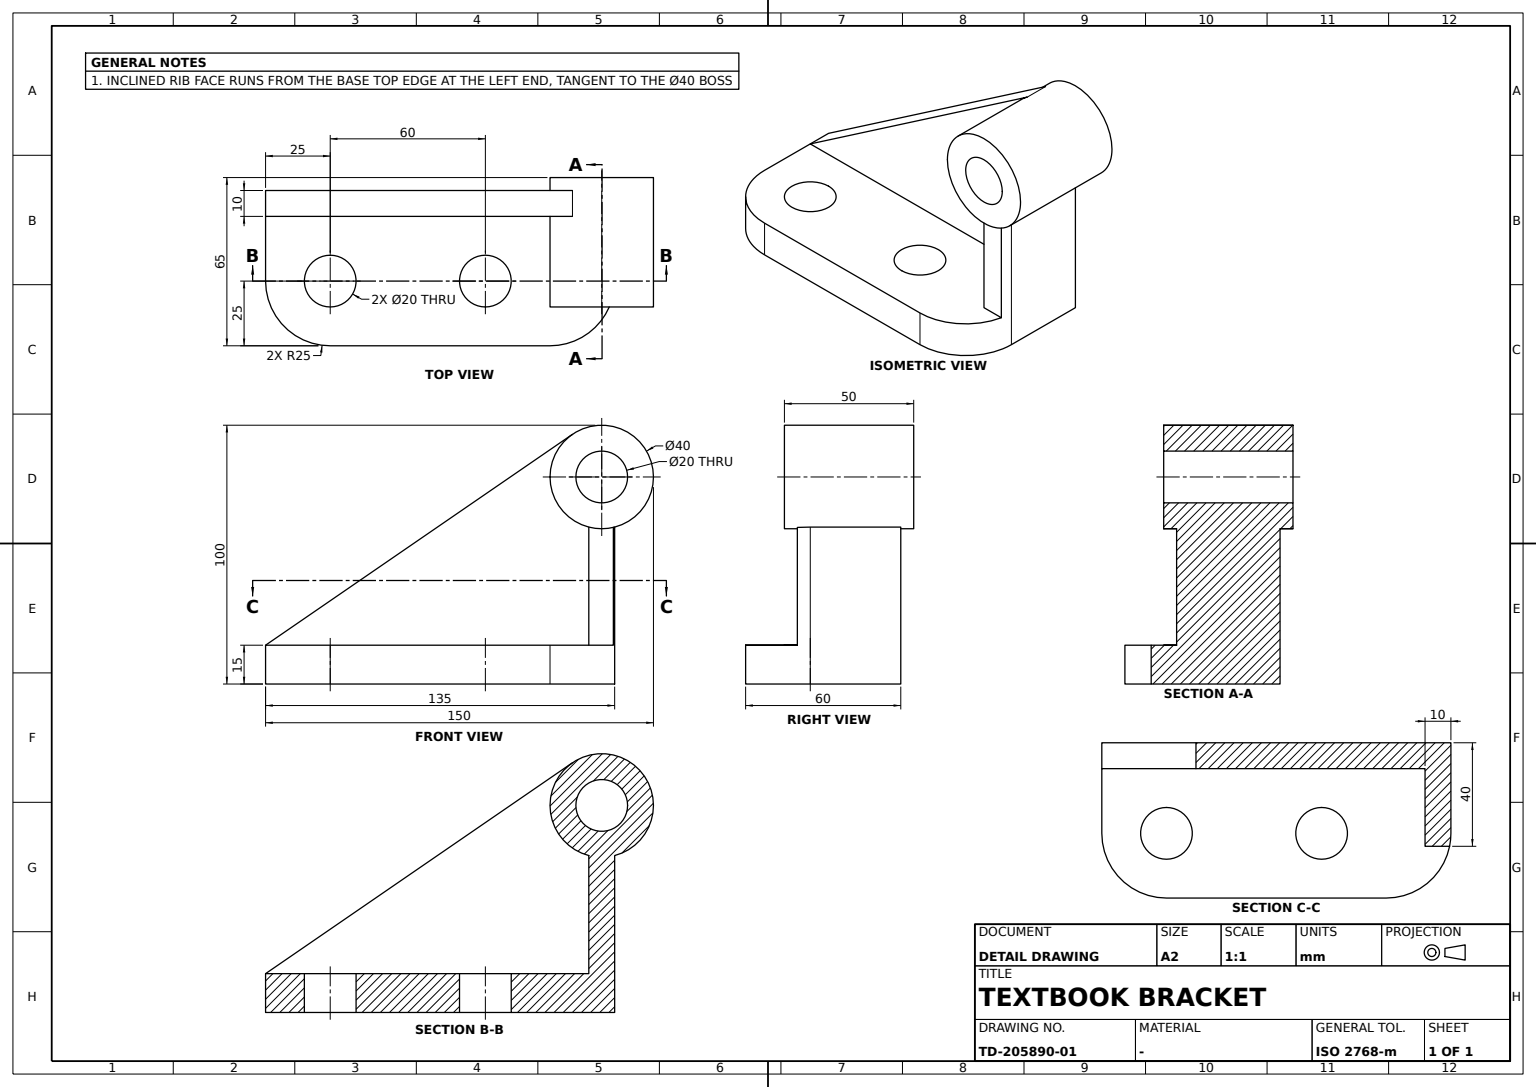
ISO-10303-21;
HEADER;
FILE_DESCRIPTION((''),'2;1');
FILE_NAME('','',(''),(''),'','','');
FILE_SCHEMA(('AUTOMOTIVE_DESIGN'));
ENDSEC;
DATA;
#1=APPLICATION_CONTEXT('');
#2=PRODUCT_CONTEXT('',#1,'mechanical');
#3=PRODUCT('','','',(#2));
#4=PRODUCT_DEFINITION_FORMATION('','',#3);
#5=PRODUCT_DEFINITION_CONTEXT('',#1,'design');
#6=PRODUCT_DEFINITION('','',#4,#5);
#7=PRODUCT_DEFINITION_SHAPE('','',#6);
#8=(LENGTH_UNIT()NAMED_UNIT(*)SI_UNIT(.MILLI.,.METRE.));
#9=(NAMED_UNIT(*)PLANE_ANGLE_UNIT()SI_UNIT($,.RADIAN.));
#10=(NAMED_UNIT(*)SI_UNIT($,.STERADIAN.)SOLID_ANGLE_UNIT());
#11=UNCERTAINTY_MEASURE_WITH_UNIT(LENGTH_MEASURE(1.E-05),#8,'distance_accuracy_value','');
#12=(GEOMETRIC_REPRESENTATION_CONTEXT(3)GLOBAL_UNCERTAINTY_ASSIGNED_CONTEXT((#11))GLOBAL_UNIT_ASSIGNED_CONTEXT((#8,#9,#10))REPRESENTATION_CONTEXT('',''));
#13=CARTESIAN_POINT('',(10.,55.,80.));
#14=VERTEX_POINT('',#13);
#15=CARTESIAN_POINT('',(10.,70.,60.635083));
#16=VERTEX_POINT('',#15);
#17=CARTESIAN_POINT('',(10.,75.,80.));
#18=DIRECTION('',(1.,0.,0.));
#19=DIRECTION('',(0.,1.,0.));
#20=AXIS2_PLACEMENT_3D('',#17,#18,#19);
#21=CIRCLE('',#20,20.);
#22=EDGE_CURVE('',#14,#16,#21,.T.);
#23=ORIENTED_EDGE('',*,*,#22,.T.);
#24=CARTESIAN_POINT('',(10.,80.,60.635083));
#25=VERTEX_POINT('',#24);
#26=EDGE_CURVE('',#16,#25,#21,.T.);
#27=ORIENTED_EDGE('',*,*,#26,.T.);
#28=CARTESIAN_POINT('',(10.,95.,80.));
#29=VERTEX_POINT('',#28);
#30=EDGE_CURVE('',#25,#29,#21,.T.);
#31=ORIENTED_EDGE('',*,*,#30,.T.);
#32=EDGE_CURVE('',#29,#14,#21,.T.);
#33=ORIENTED_EDGE('',*,*,#32,.T.);
#34=EDGE_LOOP('',(#23,#27,#31,#33));
#35=FACE_OUTER_BOUND('',#34,.T.);
#36=CARTESIAN_POINT('',(10.,85.,80.));
#37=VERTEX_POINT('',#36);
#38=CARTESIAN_POINT('',(10.,65.,80.));
#39=VERTEX_POINT('',#38);
#40=CIRCLE('',#20,10.);
#41=EDGE_CURVE('',#37,#39,#40,.T.);
#42=ORIENTED_EDGE('',*,*,#41,.F.);
#43=EDGE_CURVE('',#39,#37,#40,.T.);
#44=ORIENTED_EDGE('',*,*,#43,.F.);
#45=EDGE_LOOP('',(#42,#44));
#46=FACE_BOUND('',#45,.T.);
#47=CARTESIAN_POINT('',(10.,0.,0.));
#48=AXIS2_PLACEMENT_3D('',#47,#18,#19);
#49=PLANE('',#48);
#50=ADVANCED_FACE('',(#35,#46),#49,.T.);
#51=CARTESIAN_POINT('',(-35.,55.,80.));
#52=VERTEX_POINT('',#51);
#53=CARTESIAN_POINT('',(-40.,55.,80.));
#54=VERTEX_POINT('',#53);
#55=CARTESIAN_POINT('',(-15.,55.,80.));
#56=DIRECTION('',(-1.,0.,0.));
#57=VECTOR('',#56,1000.);
#58=LINE('',#55,#57);
#59=EDGE_CURVE('',#52,#54,#58,.T.);
#60=ORIENTED_EDGE('',*,*,#59,.F.);
#61=CARTESIAN_POINT('',(-35.,63.679274,96.487606));
#62=VERTEX_POINT('',#61);
#63=CARTESIAN_POINT('',(-35.,75.,80.));
#64=AXIS2_PLACEMENT_3D('',#63,#18,#19);
#65=CIRCLE('',#64,20.);
#66=EDGE_CURVE('',#62,#52,#65,.T.);
#67=ORIENTED_EDGE('',*,*,#66,.F.);
#68=CARTESIAN_POINT('',(-25.,63.679274,96.487606));
#69=VERTEX_POINT('',#68);
#70=CARTESIAN_POINT('',(-15.,63.679274,96.487606));
#71=VECTOR('',#18,1000.);
#72=LINE('',#70,#71);
#73=EDGE_CURVE('',#62,#69,#72,.T.);
#74=ORIENTED_EDGE('',*,*,#73,.T.);
#75=CARTESIAN_POINT('',(-25.,55.,80.));
#76=VERTEX_POINT('',#75);
#77=CARTESIAN_POINT('',(-25.,75.,80.));
#78=AXIS2_PLACEMENT_3D('',#77,#18,#19);
#79=CIRCLE('',#78,20.);
#80=EDGE_CURVE('',#69,#76,#79,.T.);
#81=ORIENTED_EDGE('',*,*,#80,.T.);
#82=EDGE_CURVE('',#14,#76,#58,.T.);
#83=ORIENTED_EDGE('',*,*,#82,.F.);
#84=ORIENTED_EDGE('',*,*,#32,.F.);
#85=CARTESIAN_POINT('',(-40.,95.,80.));
#86=VERTEX_POINT('',#85);
#87=CARTESIAN_POINT('',(-15.,95.,80.));
#88=LINE('',#87,#57);
#89=EDGE_CURVE('',#29,#86,#88,.T.);
#90=ORIENTED_EDGE('',*,*,#89,.T.);
#91=CARTESIAN_POINT('',(-40.,75.,80.));
#92=AXIS2_PLACEMENT_3D('',#91,#18,#19);
#93=CIRCLE('',#92,20.);
#94=EDGE_CURVE('',#86,#54,#93,.T.);
#95=ORIENTED_EDGE('',*,*,#94,.T.);
#96=EDGE_LOOP('',(#60,#67,#74,#81,#83,#84,#90,#95));
#97=FACE_OUTER_BOUND('',#96,.T.);
#98=CARTESIAN_POINT('',(-15.,75.,80.));
#99=AXIS2_PLACEMENT_3D('',#98,#56,#19);
#100=CYLINDRICAL_SURFACE('',#99,20.);
#101=ADVANCED_FACE('',(#97),#100,.T.);
#102=CARTESIAN_POINT('',(0.,-55.,0.));
#103=VERTEX_POINT('',#102);
#104=CARTESIAN_POINT('',(25.,-30.,0.));
#105=VERTEX_POINT('',#104);
#106=CARTESIAN_POINT('',(0.,-30.,0.));
#107=DIRECTION('',(0.,0.,1.));
#108=AXIS2_PLACEMENT_3D('',#106,#107,#56);
#109=CIRCLE('',#108,25.);
#110=EDGE_CURVE('',#103,#105,#109,.T.);
#111=ORIENTED_EDGE('',*,*,#110,.T.);
#112=CARTESIAN_POINT('',(25.,-30.,15.));
#113=VERTEX_POINT('',#112);
#114=CARTESIAN_POINT('',(25.,-30.,7.5));
#115=VECTOR('',#107,1000.);
#116=LINE('',#114,#115);
#117=EDGE_CURVE('',#105,#113,#116,.T.);
#118=ORIENTED_EDGE('',*,*,#117,.T.);
#119=CARTESIAN_POINT('',(0.,-55.,15.));
#120=VERTEX_POINT('',#119);
#121=CARTESIAN_POINT('',(0.,-30.,15.));
#122=DIRECTION('',(0.,0.,-1.));
#123=AXIS2_PLACEMENT_3D('',#121,#122,#56);
#124=CIRCLE('',#123,25.);
#125=EDGE_CURVE('',#113,#120,#124,.T.);
#126=ORIENTED_EDGE('',*,*,#125,.T.);
#127=CARTESIAN_POINT('',(0.,-55.,7.5));
#128=LINE('',#127,#115);
#129=EDGE_CURVE('',#103,#120,#128,.T.);
#130=ORIENTED_EDGE('',*,*,#129,.F.);
#131=EDGE_LOOP('',(#111,#118,#126,#130));
#132=FACE_OUTER_BOUND('',#131,.T.);
#133=CARTESIAN_POINT('',(0.,-30.,7.5));
#134=AXIS2_PLACEMENT_3D('',#133,#122,#18);
#135=CYLINDRICAL_SURFACE('',#134,25.);
#136=ADVANCED_FACE('',(#132),#135,.T.);
#137=CARTESIAN_POINT('',(-40.,65.,80.));
#138=VERTEX_POINT('',#137);
#139=CARTESIAN_POINT('',(-40.,85.,80.));
#140=VERTEX_POINT('',#139);
#141=CIRCLE('',#92,10.);
#142=EDGE_CURVE('',#138,#140,#141,.T.);
#143=ORIENTED_EDGE('',*,*,#142,.F.);
#144=CARTESIAN_POINT('',(-15.,65.,80.));
#145=LINE('',#144,#71);
#146=EDGE_CURVE('',#138,#39,#145,.T.);
#147=ORIENTED_EDGE('',*,*,#146,.T.);
#148=ORIENTED_EDGE('',*,*,#43,.T.);
#149=CARTESIAN_POINT('',(-15.,85.,80.));
#150=LINE('',#149,#71);
#151=EDGE_CURVE('',#140,#37,#150,.T.);
#152=ORIENTED_EDGE('',*,*,#151,.F.);
#153=EDGE_LOOP('',(#143,#147,#148,#152));
#154=FACE_OUTER_BOUND('',#153,.T.);
#155=CYLINDRICAL_SURFACE('',#99,10.);
#156=ADVANCED_FACE('',(#154),#155,.F.);
#157=CARTESIAN_POINT('',(5.,70.,15.));
#158=VERTEX_POINT('',#157);
#159=CARTESIAN_POINT('',(5.,79.494897,15.));
#160=VERTEX_POINT('',#159);
#161=CARTESIAN_POINT('',(5.,74.747449,15.));
#162=VECTOR('',#19,1000.);
#163=LINE('',#161,#162);
#164=EDGE_CURVE('',#158,#160,#163,.T.);
#165=ORIENTED_EDGE('',*,*,#164,.T.);
#166=CARTESIAN_POINT('',(5.,79.494897,60.511647));
#167=VERTEX_POINT('',#166);
#168=CARTESIAN_POINT('',(5.,79.494897,37.755824));
#169=VECTOR('',#122,1000.);
#170=LINE('',#168,#169);
#171=EDGE_CURVE('',#167,#160,#170,.T.);
#172=ORIENTED_EDGE('',*,*,#171,.F.);
#173=CARTESIAN_POINT('',(5.,70.,60.635083));
#174=VERTEX_POINT('',#173);
#175=CARTESIAN_POINT('',(5.,75.,80.));
#176=AXIS2_PLACEMENT_3D('',#175,#18,#19);
#177=CIRCLE('',#176,20.);
#178=EDGE_CURVE('',#174,#167,#177,.T.);
#179=ORIENTED_EDGE('',*,*,#178,.F.);
#180=CARTESIAN_POINT('',(5.,70.,37.817542));
#181=LINE('',#180,#169);
#182=EDGE_CURVE('',#174,#158,#181,.T.);
#183=ORIENTED_EDGE('',*,*,#182,.T.);
#184=EDGE_LOOP('',(#165,#172,#179,#183));
#185=FACE_OUTER_BOUND('',#184,.T.);
#186=CARTESIAN_POINT('',(5.,0.,0.));
#187=AXIS2_PLACEMENT_3D('',#186,#18,#19);
#188=PLANE('',#187);
#189=ADVANCED_FACE('',(#185),#188,.T.);
#190=CARTESIAN_POINT('',(-35.,-55.,15.));
#191=VERTEX_POINT('',#190);
#192=CARTESIAN_POINT('',(-35.,4.339637,55.743803));
#193=DIRECTION('',(0.,-0.824380311,-0.566036309));
#194=VECTOR('',#193,1000.);
#195=LINE('',#192,#194);
#196=EDGE_CURVE('',#62,#191,#195,.T.);
#197=ORIENTED_EDGE('',*,*,#196,.T.);
#198=CARTESIAN_POINT('',(-25.,-55.,15.));
#199=VERTEX_POINT('',#198);
#200=CARTESIAN_POINT('',(-30.,-55.,15.));
#201=LINE('',#200,#71);
#202=EDGE_CURVE('',#191,#199,#201,.T.);
#203=ORIENTED_EDGE('',*,*,#202,.T.);
#204=CARTESIAN_POINT('',(-25.,4.339637,55.743803));
#205=LINE('',#204,#194);
#206=EDGE_CURVE('',#69,#199,#205,.T.);
#207=ORIENTED_EDGE('',*,*,#206,.F.);
#208=ORIENTED_EDGE('',*,*,#73,.F.);
#209=EDGE_LOOP('',(#197,#203,#207,#208));
#210=FACE_OUTER_BOUND('',#209,.T.);
#211=DIRECTION('',(0.,0.566036309,-0.824380311));
#212=DIRECTION('',(0.,0.824380311,0.566036309));
#213=AXIS2_PLACEMENT_3D('',#61,#211,#212);
#214=PLANE('',#213);
#215=ADVANCED_FACE('',(#210),#214,.F.);
#216=ORIENTED_EDGE('',*,*,#66,.T.);
#217=CARTESIAN_POINT('',(-35.,70.,60.635083));
#218=VERTEX_POINT('',#217);
#219=EDGE_CURVE('',#52,#218,#65,.T.);
#220=ORIENTED_EDGE('',*,*,#219,.T.);
#221=CARTESIAN_POINT('',(-35.,80.,60.635083));
#222=VERTEX_POINT('',#221);
#223=EDGE_CURVE('',#218,#222,#65,.T.);
#224=ORIENTED_EDGE('',*,*,#223,.T.);
#225=CARTESIAN_POINT('',(-35.,80.,0.));
#226=VERTEX_POINT('',#225);
#227=CARTESIAN_POINT('',(-35.,80.,30.317542));
#228=LINE('',#227,#115);
#229=EDGE_CURVE('',#226,#222,#228,.T.);
#230=ORIENTED_EDGE('',*,*,#229,.F.);
#231=CARTESIAN_POINT('',(-35.,-55.,0.));
#232=VERTEX_POINT('',#231);
#233=CARTESIAN_POINT('',(-35.,12.5,0.));
#234=DIRECTION('',(0.,-1.,0.));
#235=VECTOR('',#234,1000.);
#236=LINE('',#233,#235);
#237=EDGE_CURVE('',#226,#232,#236,.T.);
#238=ORIENTED_EDGE('',*,*,#237,.T.);
#239=CARTESIAN_POINT('',(-35.,-55.,7.5));
#240=LINE('',#239,#169);
#241=EDGE_CURVE('',#191,#232,#240,.T.);
#242=ORIENTED_EDGE('',*,*,#241,.F.);
#243=ORIENTED_EDGE('',*,*,#196,.F.);
#244=EDGE_LOOP('',(#216,#220,#224,#230,#238,#242,#243));
#245=FACE_OUTER_BOUND('',#244,.T.);
#246=CARTESIAN_POINT('',(-35.,0.,0.));
#247=AXIS2_PLACEMENT_3D('',#246,#18,#19);
#248=PLANE('',#247);
#249=ADVANCED_FACE('',(#245),#248,.F.);
#250=CARTESIAN_POINT('',(10.,30.,0.));
#251=VERTEX_POINT('',#250);
#252=CARTESIAN_POINT('',(-10.,30.,0.));
#253=VERTEX_POINT('',#252);
#254=CARTESIAN_POINT('',(0.,30.,0.));
#255=AXIS2_PLACEMENT_3D('',#254,#107,#56);
#256=CIRCLE('',#255,10.);
#257=EDGE_CURVE('',#251,#253,#256,.T.);
#258=ORIENTED_EDGE('',*,*,#257,.T.);
#259=EDGE_CURVE('',#253,#251,#256,.T.);
#260=ORIENTED_EDGE('',*,*,#259,.T.);
#261=EDGE_LOOP('',(#258,#260));
#262=FACE_BOUND('',#261,.T.);
#263=CARTESIAN_POINT('',(-17.5,-55.,0.));
#264=LINE('',#263,#71);
#265=EDGE_CURVE('',#232,#103,#264,.T.);
#266=ORIENTED_EDGE('',*,*,#265,.F.);
#267=ORIENTED_EDGE('',*,*,#237,.F.);
#268=CARTESIAN_POINT('',(0.,80.,0.));
#269=VERTEX_POINT('',#268);
#270=CARTESIAN_POINT('',(-17.5,80.,0.));
#271=LINE('',#270,#57);
#272=EDGE_CURVE('',#269,#226,#271,.T.);
#273=ORIENTED_EDGE('',*,*,#272,.F.);
#274=CARTESIAN_POINT('',(25.,55.,0.));
#275=VERTEX_POINT('',#274);
#276=CARTESIAN_POINT('',(0.,55.,0.));
#277=AXIS2_PLACEMENT_3D('',#276,#107,#56);
#278=CIRCLE('',#277,25.);
#279=EDGE_CURVE('',#275,#269,#278,.T.);
#280=ORIENTED_EDGE('',*,*,#279,.F.);
#281=CARTESIAN_POINT('',(25.,12.5,0.));
#282=LINE('',#281,#162);
#283=EDGE_CURVE('',#105,#275,#282,.T.);
#284=ORIENTED_EDGE('',*,*,#283,.F.);
#285=ORIENTED_EDGE('',*,*,#110,.F.);
#286=EDGE_LOOP('',(#266,#267,#273,#280,#284,#285));
#287=FACE_OUTER_BOUND('',#286,.T.);
#288=CARTESIAN_POINT('',(10.,-30.,0.));
#289=VERTEX_POINT('',#288);
#290=CARTESIAN_POINT('',(-10.,-30.,0.));
#291=VERTEX_POINT('',#290);
#292=CIRCLE('',#108,10.);
#293=EDGE_CURVE('',#289,#291,#292,.T.);
#294=ORIENTED_EDGE('',*,*,#293,.T.);
#295=EDGE_CURVE('',#291,#289,#292,.T.);
#296=ORIENTED_EDGE('',*,*,#295,.T.);
#297=EDGE_LOOP('',(#294,#296));
#298=FACE_BOUND('',#297,.T.);
#299=CARTESIAN_POINT('',(0.,0.,0.));
#300=AXIS2_PLACEMENT_3D('',#299,#107,#56);
#301=PLANE('',#300);
#302=ADVANCED_FACE('',(#262,#287,#298),#301,.F.);
#303=CARTESIAN_POINT('',(25.,55.,15.));
#304=VERTEX_POINT('',#303);
#305=CARTESIAN_POINT('',(25.,12.5,15.));
#306=LINE('',#305,#162);
#307=EDGE_CURVE('',#113,#304,#306,.T.);
#308=ORIENTED_EDGE('',*,*,#307,.F.);
#309=ORIENTED_EDGE('',*,*,#117,.F.);
#310=ORIENTED_EDGE('',*,*,#283,.T.);
#311=CARTESIAN_POINT('',(25.,55.,7.5));
#312=LINE('',#311,#115);
#313=EDGE_CURVE('',#275,#304,#312,.T.);
#314=ORIENTED_EDGE('',*,*,#313,.T.);
#315=EDGE_LOOP('',(#308,#309,#310,#314));
#316=FACE_OUTER_BOUND('',#315,.T.);
#317=CARTESIAN_POINT('',(25.,-55.,0.));
#318=AXIS2_PLACEMENT_3D('',#317,#18,#19);
#319=PLANE('',#318);
#320=ADVANCED_FACE('',(#316),#319,.T.);
#321=CARTESIAN_POINT('',(-10.,-30.,15.));
#322=VERTEX_POINT('',#321);
#323=CARTESIAN_POINT('',(10.,-30.,15.));
#324=VERTEX_POINT('',#323);
#325=AXIS2_PLACEMENT_3D('',#121,#107,#56);
#326=CIRCLE('',#325,10.);
#327=EDGE_CURVE('',#322,#324,#326,.T.);
#328=ORIENTED_EDGE('',*,*,#327,.T.);
#329=CARTESIAN_POINT('',(10.,-30.,7.5));
#330=LINE('',#329,#115);
#331=EDGE_CURVE('',#289,#324,#330,.T.);
#332=ORIENTED_EDGE('',*,*,#331,.F.);
#333=ORIENTED_EDGE('',*,*,#295,.F.);
#334=CARTESIAN_POINT('',(-10.,-30.,7.5));
#335=LINE('',#334,#115);
#336=EDGE_CURVE('',#291,#322,#335,.T.);
#337=ORIENTED_EDGE('',*,*,#336,.T.);
#338=EDGE_LOOP('',(#328,#332,#333,#337));
#339=FACE_OUTER_BOUND('',#338,.T.);
#340=AXIS2_PLACEMENT_3D('',#133,#122,#56);
#341=CYLINDRICAL_SURFACE('',#340,10.);
#342=ADVANCED_FACE('',(#339),#341,.F.);
#343=ORIENTED_EDGE('',*,*,#259,.F.);
#344=CARTESIAN_POINT('',(-10.,30.,15.));
#345=VERTEX_POINT('',#344);
#346=CARTESIAN_POINT('',(-10.,30.,7.5));
#347=LINE('',#346,#115);
#348=EDGE_CURVE('',#253,#345,#347,.T.);
#349=ORIENTED_EDGE('',*,*,#348,.T.);
#350=CARTESIAN_POINT('',(10.,30.,15.));
#351=VERTEX_POINT('',#350);
#352=CARTESIAN_POINT('',(0.,30.,15.));
#353=AXIS2_PLACEMENT_3D('',#352,#107,#56);
#354=CIRCLE('',#353,10.);
#355=EDGE_CURVE('',#345,#351,#354,.T.);
#356=ORIENTED_EDGE('',*,*,#355,.T.);
#357=CARTESIAN_POINT('',(10.,30.,7.5));
#358=LINE('',#357,#115);
#359=EDGE_CURVE('',#251,#351,#358,.T.);
#360=ORIENTED_EDGE('',*,*,#359,.F.);
#361=EDGE_LOOP('',(#343,#349,#356,#360));
#362=FACE_OUTER_BOUND('',#361,.T.);
#363=CARTESIAN_POINT('',(0.,30.,7.5));
#364=AXIS2_PLACEMENT_3D('',#363,#122,#56);
#365=CYLINDRICAL_SURFACE('',#364,10.);
#366=ADVANCED_FACE('',(#362),#365,.F.);
#367=CARTESIAN_POINT('',(-12.5,-55.,15.));
#368=LINE('',#367,#71);
#369=EDGE_CURVE('',#199,#120,#368,.T.);
#370=ORIENTED_EDGE('',*,*,#369,.F.);
#371=ORIENTED_EDGE('',*,*,#202,.F.);
#372=ORIENTED_EDGE('',*,*,#241,.T.);
#373=ORIENTED_EDGE('',*,*,#265,.T.);
#374=ORIENTED_EDGE('',*,*,#129,.T.);
#375=EDGE_LOOP('',(#370,#371,#372,#373,#374));
#376=FACE_OUTER_BOUND('',#375,.T.);
#377=CARTESIAN_POINT('',(-25.,-55.,0.));
#378=AXIS2_PLACEMENT_3D('',#377,#234,#18);
#379=PLANE('',#378);
#380=ADVANCED_FACE('',(#376),#379,.T.);
#381=CARTESIAN_POINT('',(-40.,70.,60.635083));
#382=VERTEX_POINT('',#381);
#383=CARTESIAN_POINT('',(-15.,70.,60.635083));
#384=LINE('',#383,#71);
#385=EDGE_CURVE('',#382,#218,#384,.T.);
#386=ORIENTED_EDGE('',*,*,#385,.T.);
#387=ORIENTED_EDGE('',*,*,#219,.F.);
#388=ORIENTED_EDGE('',*,*,#59,.T.);
#389=EDGE_CURVE('',#54,#382,#93,.T.);
#390=ORIENTED_EDGE('',*,*,#389,.T.);
#391=EDGE_LOOP('',(#386,#387,#388,#390));
#392=FACE_OUTER_BOUND('',#391,.T.);
#393=ADVANCED_FACE('',(#392),#100,.T.);
#394=ORIENTED_EDGE('',*,*,#331,.T.);
#395=EDGE_CURVE('',#324,#322,#326,.T.);
#396=ORIENTED_EDGE('',*,*,#395,.T.);
#397=ORIENTED_EDGE('',*,*,#336,.F.);
#398=ORIENTED_EDGE('',*,*,#293,.F.);
#399=EDGE_LOOP('',(#394,#396,#397,#398));
#400=FACE_OUTER_BOUND('',#399,.T.);
#401=ADVANCED_FACE('',(#400),#341,.F.);
#402=ORIENTED_EDGE('',*,*,#182,.F.);
#403=CARTESIAN_POINT('',(-25.,70.,60.635083));
#404=VERTEX_POINT('',#403);
#405=CARTESIAN_POINT('',(-10.,70.,60.635083));
#406=LINE('',#405,#71);
#407=EDGE_CURVE('',#404,#174,#406,.T.);
#408=ORIENTED_EDGE('',*,*,#407,.F.);
#409=CARTESIAN_POINT('',(-25.,70.,15.));
#410=VERTEX_POINT('',#409);
#411=CARTESIAN_POINT('',(-25.,70.,37.817542));
#412=LINE('',#411,#115);
#413=EDGE_CURVE('',#410,#404,#412,.T.);
#414=ORIENTED_EDGE('',*,*,#413,.F.);
#415=CARTESIAN_POINT('',(-10.,70.,15.));
#416=LINE('',#415,#71);
#417=EDGE_CURVE('',#410,#158,#416,.T.);
#418=ORIENTED_EDGE('',*,*,#417,.T.);
#419=EDGE_LOOP('',(#402,#408,#414,#418));
#420=FACE_OUTER_BOUND('',#419,.T.);
#421=CARTESIAN_POINT('',(-35.,70.,15.));
#422=AXIS2_PLACEMENT_3D('',#421,#19,#107);
#423=PLANE('',#422);
#424=ADVANCED_FACE('',(#420),#423,.F.);
#425=ORIENTED_EDGE('',*,*,#413,.T.);
#426=EDGE_CURVE('',#76,#404,#79,.T.);
#427=ORIENTED_EDGE('',*,*,#426,.F.);
#428=ORIENTED_EDGE('',*,*,#80,.F.);
#429=ORIENTED_EDGE('',*,*,#206,.T.);
#430=CARTESIAN_POINT('',(-25.,7.5,15.));
#431=LINE('',#430,#162);
#432=EDGE_CURVE('',#199,#410,#431,.T.);
#433=ORIENTED_EDGE('',*,*,#432,.T.);
#434=EDGE_LOOP('',(#425,#427,#428,#429,#433));
#435=FACE_OUTER_BOUND('',#434,.T.);
#436=CARTESIAN_POINT('',(-25.,0.,0.));
#437=AXIS2_PLACEMENT_3D('',#436,#18,#19);
#438=PLANE('',#437);
#439=ADVANCED_FACE('',(#435),#438,.T.);
#440=EDGE_CURVE('',#351,#345,#354,.T.);
#441=ORIENTED_EDGE('',*,*,#440,.T.);
#442=ORIENTED_EDGE('',*,*,#348,.F.);
#443=ORIENTED_EDGE('',*,*,#257,.F.);
#444=ORIENTED_EDGE('',*,*,#359,.T.);
#445=EDGE_LOOP('',(#441,#442,#443,#444));
#446=FACE_OUTER_BOUND('',#445,.T.);
#447=ADVANCED_FACE('',(#446),#365,.F.);
#448=CARTESIAN_POINT('',(0.,80.,60.635083));
#449=VERTEX_POINT('',#448);
#450=CARTESIAN_POINT('',(-15.,80.,60.635083));
#451=LINE('',#450,#71);
#452=EDGE_CURVE('',#449,#25,#451,.T.);
#453=ORIENTED_EDGE('',*,*,#452,.T.);
#454=ORIENTED_EDGE('',*,*,#26,.F.);
#455=EDGE_CURVE('',#174,#16,#384,.T.);
#456=ORIENTED_EDGE('',*,*,#455,.F.);
#457=ORIENTED_EDGE('',*,*,#178,.T.);
#458=CARTESIAN_POINT('',(1.259002,80.,60.635083));
#459=CARTESIAN_POINT('',(2.517984,79.91545,60.613232));
#460=CARTESIAN_POINT('',(3.767745,79.74643,60.569662));
#461=B_SPLINE_CURVE_WITH_KNOTS('',4,(#448,#458,#459,#460,#166),.UNSPECIFIED.,.F.,.F.,(5,5),(0.,7.121993344),.UNSPECIFIED.);
#462=EDGE_CURVE('',#449,#167,#461,.T.);
#463=ORIENTED_EDGE('',*,*,#462,.F.);
#464=EDGE_LOOP('',(#453,#454,#456,#457,#463));
#465=FACE_OUTER_BOUND('',#464,.T.);
#466=ADVANCED_FACE('',(#465),#100,.T.);
#467=ORIENTED_EDGE('',*,*,#30,.F.);
#468=ORIENTED_EDGE('',*,*,#452,.F.);
#469=CARTESIAN_POINT('',(-17.5,80.,60.635083));
#470=LINE('',#469,#71);
#471=EDGE_CURVE('',#222,#449,#470,.T.);
#472=ORIENTED_EDGE('',*,*,#471,.F.);
#473=CARTESIAN_POINT('',(-40.,80.,60.635083));
#474=VERTEX_POINT('',#473);
#475=EDGE_CURVE('',#474,#222,#451,.T.);
#476=ORIENTED_EDGE('',*,*,#475,.F.);
#477=EDGE_CURVE('',#474,#86,#93,.T.);
#478=ORIENTED_EDGE('',*,*,#477,.T.);
#479=ORIENTED_EDGE('',*,*,#89,.F.);
#480=EDGE_LOOP('',(#467,#468,#472,#476,#478,#479));
#481=FACE_OUTER_BOUND('',#480,.T.);
#482=ADVANCED_FACE('',(#481),#100,.T.);
#483=CARTESIAN_POINT('',(0.,80.,30.317542));
#484=LINE('',#483,#115);
#485=EDGE_CURVE('',#269,#449,#484,.T.);
#486=ORIENTED_EDGE('',*,*,#485,.F.);
#487=ORIENTED_EDGE('',*,*,#272,.T.);
#488=ORIENTED_EDGE('',*,*,#229,.T.);
#489=ORIENTED_EDGE('',*,*,#471,.T.);
#490=EDGE_LOOP('',(#486,#487,#488,#489));
#491=FACE_OUTER_BOUND('',#490,.T.);
#492=CARTESIAN_POINT('',(25.,80.,0.));
#493=AXIS2_PLACEMENT_3D('',#492,#19,#56);
#494=PLANE('',#493);
#495=ADVANCED_FACE('',(#491),#494,.T.);
#496=ORIENTED_EDGE('',*,*,#440,.F.);
#497=ORIENTED_EDGE('',*,*,#355,.F.);
#498=EDGE_LOOP('',(#496,#497));
#499=FACE_BOUND('',#498,.T.);
#500=ORIENTED_EDGE('',*,*,#327,.F.);
#501=ORIENTED_EDGE('',*,*,#395,.F.);
#502=EDGE_LOOP('',(#500,#501));
#503=FACE_BOUND('',#502,.T.);
#504=CARTESIAN_POINT('',(0.,55.,15.));
#505=AXIS2_PLACEMENT_3D('',#504,#122,#56);
#506=CIRCLE('',#505,25.);
#507=EDGE_CURVE('',#160,#304,#506,.T.);
#508=ORIENTED_EDGE('',*,*,#507,.F.);
#509=ORIENTED_EDGE('',*,*,#164,.F.);
#510=ORIENTED_EDGE('',*,*,#417,.F.);
#511=ORIENTED_EDGE('',*,*,#432,.F.);
#512=ORIENTED_EDGE('',*,*,#369,.T.);
#513=ORIENTED_EDGE('',*,*,#125,.F.);
#514=ORIENTED_EDGE('',*,*,#307,.T.);
#515=EDGE_LOOP('',(#508,#509,#510,#511,#512,#513,#514));
#516=FACE_OUTER_BOUND('',#515,.T.);
#517=CARTESIAN_POINT('',(0.,0.,15.));
#518=AXIS2_PLACEMENT_3D('',#517,#107,#56);
#519=PLANE('',#518);
#520=ADVANCED_FACE('',(#499,#503,#516),#519,.T.);
#521=ORIENTED_EDGE('',*,*,#455,.T.);
#522=ORIENTED_EDGE('',*,*,#22,.F.);
#523=ORIENTED_EDGE('',*,*,#82,.T.);
#524=ORIENTED_EDGE('',*,*,#426,.T.);
#525=ORIENTED_EDGE('',*,*,#407,.T.);
#526=EDGE_LOOP('',(#521,#522,#523,#524,#525));
#527=FACE_OUTER_BOUND('',#526,.T.);
#528=ADVANCED_FACE('',(#527),#100,.T.);
#529=ORIENTED_EDGE('',*,*,#313,.F.);
#530=ORIENTED_EDGE('',*,*,#279,.T.);
#531=ORIENTED_EDGE('',*,*,#485,.T.);
#532=ORIENTED_EDGE('',*,*,#462,.T.);
#533=ORIENTED_EDGE('',*,*,#171,.T.);
#534=ORIENTED_EDGE('',*,*,#507,.T.);
#535=EDGE_LOOP('',(#529,#530,#531,#532,#533,#534));
#536=FACE_OUTER_BOUND('',#535,.T.);
#537=CARTESIAN_POINT('',(0.,55.,30.317542));
#538=AXIS2_PLACEMENT_3D('',#537,#122,#19);
#539=CYLINDRICAL_SURFACE('',#538,25.);
#540=ADVANCED_FACE('',(#536),#539,.T.);
#541=ORIENTED_EDGE('',*,*,#146,.F.);
#542=EDGE_CURVE('',#140,#138,#141,.T.);
#543=ORIENTED_EDGE('',*,*,#542,.F.);
#544=ORIENTED_EDGE('',*,*,#151,.T.);
#545=ORIENTED_EDGE('',*,*,#41,.T.);
#546=EDGE_LOOP('',(#541,#543,#544,#545));
#547=FACE_OUTER_BOUND('',#546,.T.);
#548=ADVANCED_FACE('',(#547),#155,.F.);
#549=ORIENTED_EDGE('',*,*,#475,.T.);
#550=ORIENTED_EDGE('',*,*,#223,.F.);
#551=ORIENTED_EDGE('',*,*,#385,.F.);
#552=EDGE_CURVE('',#382,#474,#93,.T.);
#553=ORIENTED_EDGE('',*,*,#552,.T.);
#554=EDGE_LOOP('',(#549,#550,#551,#553));
#555=FACE_OUTER_BOUND('',#554,.T.);
#556=ADVANCED_FACE('',(#555),#100,.T.);
#557=ORIENTED_EDGE('',*,*,#542,.T.);
#558=ORIENTED_EDGE('',*,*,#142,.T.);
#559=EDGE_LOOP('',(#557,#558));
#560=FACE_BOUND('',#559,.T.);
#561=ORIENTED_EDGE('',*,*,#552,.F.);
#562=ORIENTED_EDGE('',*,*,#389,.F.);
#563=ORIENTED_EDGE('',*,*,#94,.F.);
#564=ORIENTED_EDGE('',*,*,#477,.F.);
#565=EDGE_LOOP('',(#561,#562,#563,#564));
#566=FACE_OUTER_BOUND('',#565,.T.);
#567=CARTESIAN_POINT('',(-40.,0.,0.));
#568=AXIS2_PLACEMENT_3D('',#567,#18,#19);
#569=PLANE('',#568);
#570=ADVANCED_FACE('',(#560,#566),#569,.F.);
#571=CLOSED_SHELL('',(#50,#101,#136,#156,#189,#215,#249,#302,#320,#342,#366,#380,#393,#401,#424,#439,#447,#466,#482,#495,#520,#528,#540,#548,#556,#570));
#572=MANIFOLD_SOLID_BREP('',#571);
#573=ADVANCED_BREP_SHAPE_REPRESENTATION('',(#572),#12);
#574=SHAPE_DEFINITION_REPRESENTATION(#7,#573);
ENDSEC;
END-ISO-10303-21;
